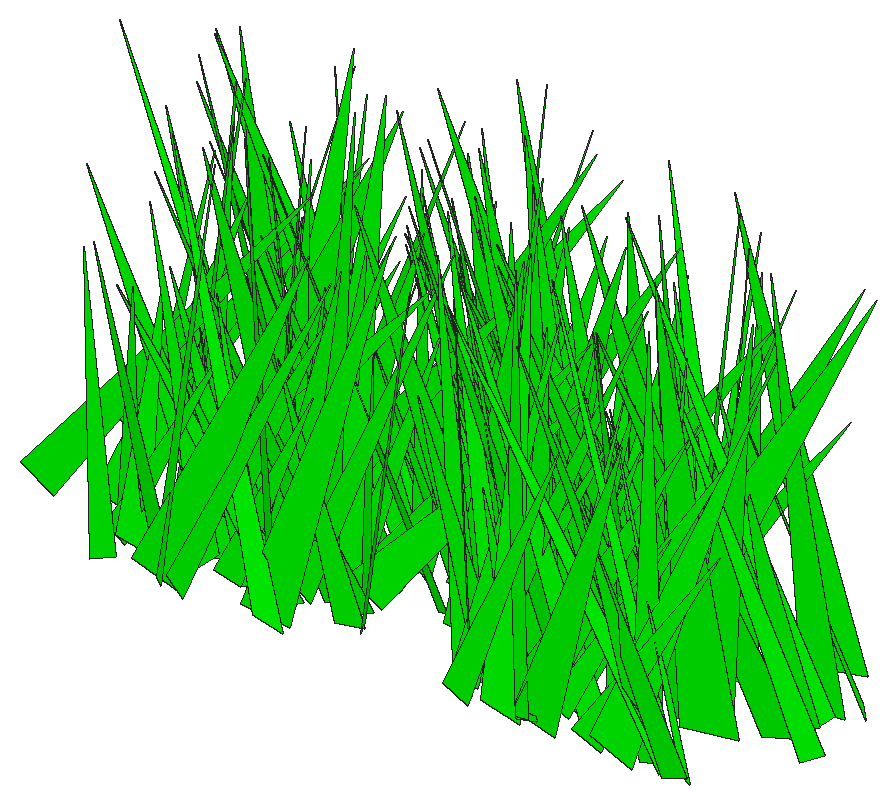
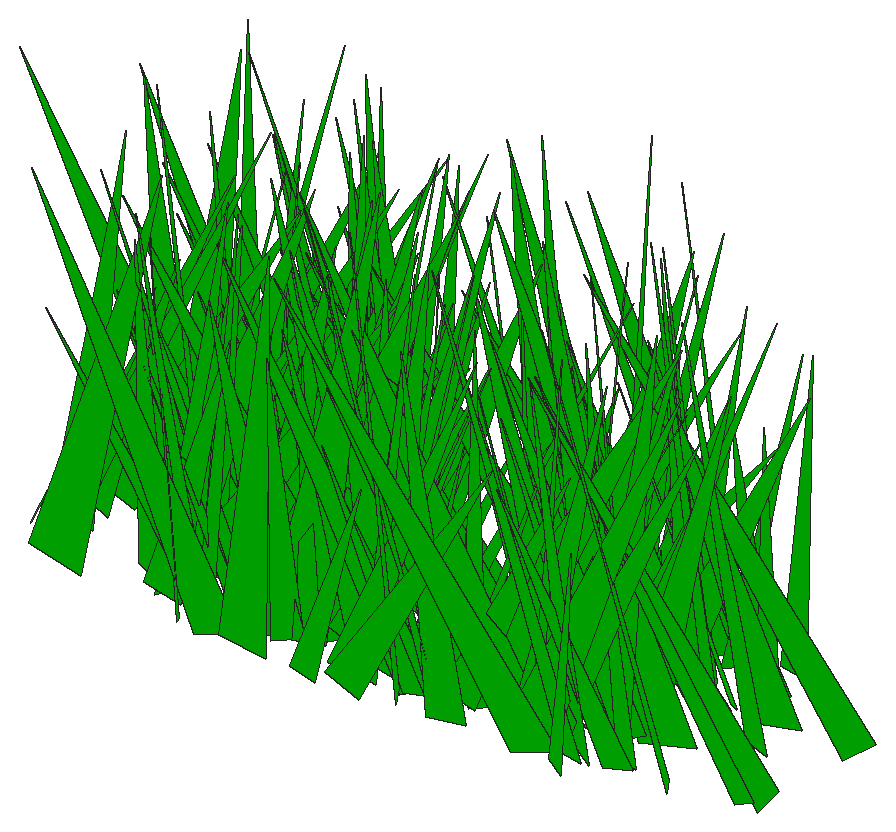
# SketchUp Ruby script. Lengths in inches.
U = 1.inch
M = Sketchup.active_model
def pt(a) = Geom::Point3d.new(a.map { |v| v * U })
def face(e, loops, mat)
  f = e.add_face(loops[0].map { |a| pt(a) })
  loops[1..].each { |l| e.add_face(l.map { |a| pt(a) }).erase! }
  f.material = f.back_material = mat if mat
  f
end
# faces: each face lists its corners as indices into pts; further lists are holes
def faces(e, pts, list, mat = nil) = list.each { |f| face(e, (f[0].is_a?(Array) ? f : [f]).map { |l| l.map { |i| pts[i] } }, mat) }
# xy, xz, yz: faces in a plane at the given z, y or x. An outline is a flat list of corners, or four numbers for a rectangle; further outlines are holes
def ring(l) = l.size == 4 ? [[l[0], l[1]], [l[2], l[1]], [l[2], l[3]], [l[0], l[3]]] : l.each_slice(2).to_a
def flat(e, list, mat, &to3) = list.each { |f| face(e, (f[0].is_a?(Array) ? f : [f]).map { |l| ring(l).map { |u, v| to3.(u, v) } }, mat) }
def xy(e, z, list, mat = nil) = flat(e, list, mat) { |x, y| [x, y, z] }
def xz(e, y, list, mat = nil) = flat(e, list, mat) { |x, z| [x, y, z] }
def yz(e, x, list, mat = nil) = flat(e, list, mat) { |y, z| [x, y, z] }
def lines(e, pts, list) = list.each { |a, b| e.add_line(pt(pts[a]), pt(pts[b])) }
# prism: a flat outline (further loops are holes) pulled along v
def prism(e, loops, v, mat = nil)
  f = face(e, loops, mat); d = Geom::Vector3d.new(v.map { |x| x * U })
  f.pushpull(f.normal.samedirection?(d) ? d.length : -d.length)
end
def box(e, o, s, mat = nil) = prism(e, [[o, [o[0] + s[0], o[1], o[2]], [o[0] + s[0], o[1] + s[1], o[2]], [o[0], o[1] + s[1], o[2]]]], [0, 0, s[2]], mat)
def at(x, y, z, deg = 0) = Geom::Transformation.translation(pt([x, y, z])) * Geom::Transformation.rotation(ORIGIN, Z_AXIS, deg.degrees)
def axes(o, x, y, z) = Geom::Transformation.new([*x, 0, *y, 0, *z, 0, *pt(o).to_a, 1])
def part(name) = M.definitions.add(name)
# library, detail: a bought-in or finely detailed component or shape, given as its bounding box
def library(name, o, s) = part(name).tap { |d| box(d.entities, o, s) }
def detail(e, o, s) = box(e.add_group.entities, o, s)
def put(e, d, t, mat = nil) = e.add_instance(d, t).tap { |i| i.material = mat if mat }
def group(e, t, mat = nil) = e.add_group.tap { |g| g.transformation = t; g.material = mat if mat }.entities
root = M.entities
M.materials.add("[0065_Lime]").color = [0, 255, 0]
c1 = part("fur_instance\#9")
p = [[0.8125,0,1.79],[0.67,-0.02,1.48],[0,-0.11,0],[0,0.11,0]]
faces(c1.entities,p,[[0,1,2,3]])
put(root,c1,axes([27.24,22.38,1.48],[7.31174,-0.39433,0.70196],[2.47884,1.00353,1.80658],[-1.57323,-0.25146,6.10893]),"[0065_Lime]")
put(root,c1,axes([31.46,23.04,1.48],[-8.52784,0.29529,1.08931],[-2.31792,-1.1863,-1.2302],[0.91482,-0.25308,7.03745]),"[0065_Lime]")
put(root,c1,axes([29,18.58,1.48],[4.59587,-0.53005,1.40933],[3.49281,0.69007,1.16069],[-2.24308,-0.01149,4.69495]),"[0065_Lime]")
put(root,c1,axes([30.38,23.19,1.48],[2.12919,0.84974,2.51321],[-6.24961,0.42319,-1.29142],[-2.65654,-0.31451,5.05242]),"[0065_Lime]")
put(root,c1,axes([28.63,20.14,1.48],[-3.00897,-0.60409,0.65925],[4.0362,-0.43666,-1.21885],[1.68757,-0.03275,4.09063]),"[0065_Lime]")
put(root,c1,axes([25.1875,24.44,1.48],[7.63571,-0.36238,0.53307],[2.54655,0.91406,-3.31261],[0.77165,0.56939,5.65715]),"[0065_Lime]")
put(root,c1,axes([31.65,20.61,1.48],[-3.71065,0.80647,0.71768],[-5.70109,-0.47805,-1.50216],[-1.10248,-0.2423,5.35235]),"[0065_Lime]")
put(root,c1,axes([25.62,24.91,1.48],[6.39063,0.54386,0.13874],[-3.71413,0.84691,1.9469],[1.10205,-0.29952,5.75696]),"[0065_Lime]")
put(root,c1,axes([32,25.42,1.48],[-3.76719,-0.84383,1.15865],[6.05294,-0.45934,1.81138],[-1.20548,0.33059,5.47439]),"[0065_Lime]")
put(root,c1,axes([29.14,19.64,1.48],[-2.3727,0.69246,0.37677],[-4.74423,-0.33875,1.09419],[1.41112,0.02545,4.31221]),"[0065_Lime]")
put(root,c1,axes([24.97,20.83,1.48],[7.30915,-0.65946,0.64194],[4.44222,0.87253,-3.43001],[1.70712,0.55304,6.17696]),"[0065_Lime]")
put(root,c1,axes([27.48,21.08,1.48],[0.90145,0.99524,0.70755],[-6.89263,0.08955,1.58951],[1.84718,-0.15155,5.58583]),"[0065_Lime]")
put(root,c1,axes([30.6,24.53,1.48],[3.62891,0.99697,2.27573],[-7.10396,0.60027,-1.31666],[-2.77481,-0.23294,6.34708]),"[0065_Lime]")
put(root,c1,axes([30.47,19.35,1.48],[-5.55156,-0.60914,0.08606],[4.02373,-0.73265,-2.03309],[1.61643,-0.2683,5.35647]),"[0065_Lime]")
put(root,c1,axes([32.46,25.47,1.48],[-4.3204,0.97206,0.76351],[-6.89822,-0.57061,-1.48346],[-1.07243,-0.24569,6.46621]),"[0065_Lime]")
put(root,c1,axes([27.8,25.44,1.48],[8.165,0.11966,1.13344],[-0.60132,1.14853,-1.19703],[-1.51831,0.18863,6.56937]),"[0065_Lime]")
put(root,c1,axes([28.43,22.59,1.48],[8.64399,-0.23036,1.70844],[1.147,1.22609,1.69991],[-2.40484,-0.24321,6.95164]),"[0065_Lime]")
put(root,c1,axes([29.45,25.125,1.48],[4.98083,-0.36586,0.65326],[2.32801,0.69361,1.27264],[-1.41576,-0.1466,4.39091]),"[0065_Lime]")
put(root,c1,axes([28.45,19.81,1.48],[3.81867,0.42883,0.98629],[-3.24796,0.45472,1.69548],[0.48393,-0.33195,3.59661]),"[0065_Lime]")
put(root,c1,axes([30.4,21.1,1.48],[6.9537,0.81374,1.27128],[-5.20212,0.98555,-2.31197],[-2.98602,0.17802,6.9883]),"[0065_Lime]")
put(root,c1,axes([31.3,20.12,1.48],[6.27949,-0.5717,1.66336],[2.93161,0.88212,2.83688],[-3.48431,-0.28814,5.38462]),"[0065_Lime]")
put(root,c1,axes([32.28,23.26,1.48],[-8.15919,-0.59671,0.88702],[3.90599,-1.13637,-1.84377],[1.99129,-0.21595,7.25112]),"[0065_Lime]")
put(root,c1,axes([30.79,26.47,1.48],[4.05133,-0.3067,0.66427],[1.45987,0.5134,2.05196],[-1.81647,-0.27143,3.13068]),"[0065_Lime]")
put(root,c1,axes([30.11,20.57,1.48],[7.8765,0.09932,2.19649],[-0.23858,1.15576,-1.18509],[-2.78109,0.18213,6.32248]),"[0065_Lime]")
put(root,c1,axes([32.36,22.14,1.48],[-3.61363,0.35537,0.74914],[-2.69143,-0.47598,-1.02391],[-0.01415,-0.21916,3.43849]),"[0065_Lime]")
put(root,c1,axes([29.12,20.96,1.48],[5.68958,-0.04407,0.13112],[0.27234,0.78178,0.98569],[-0.224,-0.16887,4.52898]),"[0065_Lime]")
put(root,c1,axes([31,25.3125,1.48],[6.60297,0.74035,0.46292],[-4.57086,0.8603,-2.9672],[-2.68159,0.35658,6.19756]),"[0065_Lime]")
put(root,c1,axes([29.42,25.52,1.48],[1.57397,0.67962,0.31538],[-4.63986,0.19407,1.3076],[1.41924,-0.11926,3.92512]),"[0065_Lime]")
put(root,c1,axes([32.07,20.42,1.48],[-4.06736,-0.10484,1.09489],[1.15393,-0.5614,1.03489],[1.01831,0.2174,3.20049]),"[0065_Lime]")
put(root,c1,axes([34.87,24.59,1.48],[-4.96476,0.99746,1.25521],[-7.07895,-0.60537,-2.40567],[-1.63042,-0.40895,6.62273]),"[0065_Lime]")
put(root,c1,axes([34.44,19.68,1.48],[-3.46979,0.62478,0.16593],[-4.0987,-0.43434,-1.9071],[-1.73542,-0.22337,4.17241]),"[0065_Lime]")
put(root,c1,axes([34.42,23.29,1.48],[-7.19379,-0.06708,0.09262],[0.49066,-0.97855,1.46741],[-0.00946,0.254,5.67783]),"[0065_Lime]")
put(root,c1,axes([32.67,25.28,1.48],[-5.43603,0.49974,2.45261],[-4.5128,-0.72754,-1.65049],[1.17224,-0.4834,5.01957]),"[0065_Lime]")
put(root,c1,axes([32.43,25.25,1.48],[7.00593,0.4856,2.47902],[-2.13062,1.03245,-2.79288],[-4.0855,0.29429,5.70761]),"[0065_Lime]")
put(root,c1,axes([33.26,19.85,1.48],[-2.34254,0.7207,0.59506],[-5.12688,-0.30624,-0.92509],[-0.74549,-0.15853,4.49218]),"[0065_Lime]")
put(root,c1,axes([32.74,21.97,1.48],[-4.70993,0.23093,0.59338],[-1.43956,-0.65652,1.0013],[1.07733,0.13233,3.93215]),"[0065_Lime]")
put(root,c1,axes([32.06,24.22,1.48],[-3.78011,-0.39336,0.58553],[2.51547,-0.52972,-1.18008],[1.42373,-0.10847,3.63959]),"[0065_Lime]")
put(root,c1,axes([30.74,18.69,1.48],[7.93736,0.22721,2.24613],[-2.16637,1.14531,1.18305],[-2.3551,-0.28777,6.48188]),"[0065_Lime]")
put(root,c1,axes([29.86,25.22,1.48],[4.81076,0.44759,1.44128],[-3.6437,0.57975,2.0139],[0.0954,-0.42761,4.23909]),"[0065_Lime]")
put(root,c1,axes([31.04,23.62,1.48],[-1.81036,1.27367,1.27731],[-9.01104,-0.29078,1.26561],[1.85082,-0.16986,7.41122]),"[0065_Lime]")
put(root,c1,axes([32,22.7,1.48],[4.61273,0.80516,0.81269],[-5.45717,0.66109,-1.45344],[-2.01241,0.05281,5.80419]),"[0065_Lime]")
put(root,c1,axes([33.73,20.03,1.48],[0.64125,-0.62776,0.59127],[4.02991,0.12615,1.59639],[-2.06071,0.05136,3.30588]),"[0065_Lime]")
put(root,c1,axes([29.18,23.7,1.48],[3.6009,-1.21002,0.8703],[8.47054,0.45484,-1.99834],[1.88317,0.26787,7.32444]),"[0065_Lime]")
put(root,c1,axes([35.4,20.51,1.48],[-6.07148,-0.63604,0.35972],[4.50379,-0.82645,1.32929],[-0.63224,0.22068,6.01489]),"[0065_Lime]")
put(root,c1,axes([32.1,21.78,1.48],[-7.56677,0.10738,3.03402],[0.73364,-1.1031,2.51875],[3.73611,0.43408,5.65023]),"[0065_Lime]")
put(root,c1,axes([32.76,20.24,1.48],[3.63636,-0.17101,1.37041],[0.25971,0.51074,1.67966],[-2.06204,-0.23724,2.62823]),"[0065_Lime]")
put(root,c1,axes([30.19,23.97,1.48],[6.06021,-0.46769,1.11053],[3.59327,0.80516,-1.61137],[-0.17445,0.33718,5.3882]),"[0065_Lime]")
put(root,c1,axes([34.64,18.52,1.48],[-8.09068,0.5651,0.45602],[-3.78052,-1.11245,1.81487],[1.4815,0.24731,7.12161]),"[0065_Lime]")
put(root,c1,axes([34.35,21.02,1.48],[0.77309,-1.23959,0.12733],[8.57589,0.11076,1.68193],[-2.07345,-0.00406,7.00399]),"[0065_Lime]")
put(root,c1,axes([33.44,19.65,1.48],[-4.9149,0.24413,1.83922],[-2.36952,-0.70189,-1.06758],[1.58637,-0.29202,4.10368]),"[0065_Lime]")
put(root,c1,axes([33.26,22.09,1.48],[-7.80588,-0.30689,2.05938],[1.01437,-1.07831,-2.84054],[3.18601,-0.40857,5.94996]),"[0065_Lime]")
put(root,c1,axes([35,23.05,1.48],[-3.42222,-0.65458,0.48968],[4.64295,-0.45558,1.0622],[-0.71087,0.17564,4.58019]),"[0065_Lime]")
put(root,c1,axes([30.7,20.7,1.48],[2.81269,-0.74102,0.40694],[5.14305,0.36296,-1.37274],[1.26841,0.17149,4.66368]),"[0065_Lime]")
put(root,c1,axes([35.09,25.21,1.48],[-1.79234,0.70766,0.99132],[-4.99689,-0.18813,-1.47738],[-1.37072,-0.23951,4.08947]),"[0065_Lime]")
put(root,c1,axes([30.75,25.83,1.48],[8.38971,-0.28534,0.46525],[1.90486,1.16624,1.24072],[-0.90679,-0.19017,6.91086]),"[0065_Lime]")
put(root,c1,axes([32.0625,21.48,1.48],[-3.36593,0.64664,1.28953],[-3.78762,-0.51809,2.16426],[3.05679,0.07008,4.10164]),"[0065_Lime]")
put(root,c1,axes([32.76,21.9375,1.48],[-3.55119,-0.59167,1.40943],[3.85319,-0.55502,-1.38384],[2.42582,0.01545,4.26138]),"[0065_Lime]")
put(root,c1,axes([30.73,18.72,1.48],[0.6966,-1.13401,1.07496],[7.68457,0.02703,-2.33927],[2.79686,0.20817,6.15959]),"[0065_Lime]")
put(root,c1,axes([29.28,21.65,1.48],[4.05134,0.88781,0.72507],[-5.68072,0.4343,3.18205],[2.90562,-0.38879,5.21019]),"[0065_Lime]")
put(root,c1,axes([32.26,19.78,1.48],[1.63236,-0.57647,0.58851],[4.05108,0.19422,-1.05954],[0.97086,0.15883,3.43162]),"[0065_Lime]")
put(root,c1,axes([32.22,24.37,1.48],[5.73566,-0.1439,0.41558],[0.83523,0.77716,1.39029],[-0.7824,-0.22528,4.53073]),"[0065_Lime]")
put(root,c1,axes([34.33,19.15,1.48],[8.27058,0.12873,3.67062],[-2.34781,1.23927,2.04372],[-3.96117,-0.46574,6.45263]),"[0065_Lime]")
put(root,c1,axes([31.28,18.66,1.48],[6.64813,0.53494,1.43953],[-4.19276,0.82237,2.57124],[0.21324,-0.50818,5.67632]),"[0065_Lime]")
put(root,c1,axes([36.32,20.58,1.48],[-3.00258,-0.41802,0.26218],[2.83445,-0.37677,1.34786],[-0.95901,0.19521,3.16287]),"[0065_Lime]")
put(root,c1,axes([33.28,20.65,1.48],[-0.06196,-0.90183,1.36953],[6.49252,-0.05703,-1.06399],[1.36816,0.22978,5.1111]),"[0065_Lime]")
put(root,c1,axes([35.7,24.1,1.48],[-4.70782,0.03814,0.87173],[-0.6939,-0.61476,-1.57809],[0.86065,-0.287,3.4961]),"[0065_Lime]")
put(root,c1,axes([33.7,22.19,1.48],[-1.936,-0.90176,1.04675],[6.26825,-0.30972,-1.27006],[1.88361,0.10383,5.30237]),"[0065_Lime]")
put(root,c1,axes([37.9,21.88,1.48],[-7.69705,-0.29198,0.29811],[2.10916,-1.07001,0.914],[0.05713,0.16589,6.42027]),"[0065_Lime]")
put(root,c1,axes([33.02,19.88,1.48],[6.88446,0.19712,0.505],[-1.12008,0.91997,-1.93019],[-1.04823,0.3116,5.37917]),"[0065_Lime]")
put(root,c1,axes([34.2,21.69,1.48],[-2.10637,1.236,2.23685],[-9.03041,-0.35594,0.96409],[1.83965,-0.33201,7.29366]),"[0065_Lime]")
put(root,c1,axes([33.24,22.75,1.48],[3.38714,-0.85288,1.06915],[6.19585,0.44979,-0.96411],[0.42222,0.24152,5.57096]),"[0065_Lime]")
put(root,c1,axes([34.39,21.06,1.48],[6.86662,0.71639,3.21811],[-6.01518,1.00453,0.99876],[-2.33711,-0.4806,6.88451]),"[0065_Lime]")
put(root,c1,axes([36.41,19.81,1.48],[-0.62911,-0.63991,1.08982],[4.63821,-0.04245,0.93635],[-1.01024,0.20361,3.6203]),"[0065_Lime]")
put(root,c1,axes([35.74,21.29,1.48],[7.47327,0.53315,1.76455],[-2.21384,0.9824,-3.74273],[-3.76836,0.48017,5.69818]),"[0065_Lime]")
put(root,c1,axes([36.03,23.34,1.48],[6.73913,0.79277,0.67794],[-4.31233,0.827,-4.04313],[-3.73207,0.47596,5.89594]),"[0065_Lime]")
put(root,c1,axes([37.95,26.56,1.48],[-0.57662,-0.79796,0.598],[5.19884,-0.02944,2.00061],[-2.40013,0.12795,4.18977]),"[0065_Lime]")
put(root,c1,axes([34.6,26.34,1.48],[-1.28453,-0.92384,0.95227],[6.46428,-0.21406,-1.18929],[1.67579,0.11757,5.31756]),"[0065_Lime]")
put(root,c1,axes([31.73,26.18,1.48],[3.05563,1.15514,0.0185],[-7.54446,0.3927,2.83958],[3.26495,-0.17366,6.54423]),"[0065_Lime]")
put(root,c1,axes([31.77,22.54,1.48],[3.23221,-0.94446,1.44478],[6.17309,0.26332,-3.36941],[3.19737,0.44636,5.04472]),"[0065_Lime]")
put(root,c1,axes([38.33,26.04,1.48],[-5.02287,-0.71257,0.95099],[5.20003,-0.67822,1.14335],[-0.20533,0.25528,5.69209]),"[0065_Lime]")
put(root,c1,axes([34.8,21.95,1.48],[4.35896,-0.42854,1.1615],[3.3495,0.58562,-1.07677],[-0.34747,0.26922,4.19117]),"[0065_Lime]")
put(root,c1,axes([36.93,24.91,1.48],[-4.01383,-0.40934,0.21134],[2.71355,-0.54436,-1.23184],[1.09097,-0.15204,3.84147]),"[0065_Lime]")
put(root,c1,axes([34.32,18.83,1.48],[4.55432,-0.95925,1.35246],[7.01581,0.6058,-1.23355],[0.38029,0.31167,6.56015]),"[0065_Lime]")
put(root,c1,axes([32.66,25.37,1.48],[6.84505,-0.88791,0.30615],[6.19986,0.92468,-1.85185],[1.27735,0.27004,7.34777]),"[0065_Lime]")
put(root,c1,axes([38.4375,22.28,1.48],[-3.7554,-0.36263,0.77595],[2.74661,-0.48085,1.2651],[-0.16095,0.25538,3.48382]),"[0065_Lime]")
put(root,c1,axes([34.23,20.41,1.48],[6.90659,0.55604,1.07512],[-4.16845,0.93448,1.52274],[-0.1713,-0.32111,6.29304]),"[0065_Lime]")
put(root,c1,axes([34.28,25.18,1.48],[2.8761,0.66224,0.83559],[-4.53985,0.31487,1.97694],[1.62973,-0.29159,4.03242]),"[0065_Lime]")
put(root,c1,axes([37.59,25.9,1.48],[-7.39528,0.13923,2.40911],[-1.65613,-1.08179,-1.26864],[2.64781,-0.28775,5.9351]),"[0065_Lime]")
put(root,c1,axes([36.42,26.12,1.48],[8.31067,0.16513,2.38382],[-0.60758,1.22146,-1.43371],[-3.09846,0.20338,6.67502]),"[0065_Lime]")
put(root,c1,axes([37.85,25.12,1.48],[-6.1838,-0.66036,0.47822],[4.29819,-0.83955,-2.07369],[1.98911,-0.23881,5.96767]),"[0065_Lime]")
put(root,c1,axes([37.63,25.28,1.48],[4.07699,-0.9895,1.08281],[6.75053,0.6025,1.63239],[-2.40623,0.01371,6.41422]),"[0065_Lime]")
put(root,c1,axes([39.42,22.9,1.48],[-6.94626,-0.01756,0.77063],[0.58219,-0.85237,2.8212],[0.75779,0.49387,4.8965]),"[0065_Lime]")
put(root,c1,axes([39.49,24.54,1.48],[-3.32818,-0.70735,0.54631],[4.9953,-0.43563,1.23452],[-0.91533,0.19454,4.75086]),"[0065_Lime]")
put(root,c1,axes([39.5,22.09,1.48],[-0.92688,-1.08023,0.89166],[7.50309,-0.08462,1.72531],[-2.00062,0.18311,6.05746]),"[0065_Lime]")
put(root,c1,axes([35.125,26.12,1.48],[8.46546,0.27052,1.33272],[-2.19824,1.18506,1.17822],[-1.24837,-0.25231,6.96274]),"[0065_Lime]")
put(root,c1,axes([38.71,23.54,1.48],[-7.23871,-0.05482,1.49299],[0.04202,-1.0323,-1.13529],[1.87599,-0.1884,5.78628]),"[0065_Lime]")
put(root,c1,axes([36.28,23.09,1.48],[5.68248,-0.03481,1.22168],[0.85153,0.74876,-1.90566],[-1.26176,0.34854,4.21591]),"[0065_Lime]")
put(root,c1,axes([39.49,22.79,1.48],[-6.30534,-0.84975,1.88278],[6.43525,-0.87268,1.06135],[0.71748,0.3595,7.0267]),"[0065_Lime]")
put(root,c1,axes([38.09,23.95,1.48],[-4.2405,-0.1173,0.95165],[0.31347,-0.57531,-1.4521],[1.40265,-0.22607,3.20157]),"[0065_Lime]")
put(root,c1,axes([36.76,19.91,1.48],[6.71529,-0.01641,1.65695],[-0.24113,0.97131,0.96898],[-2.02609,-0.17,5.37652]),"[0065_Lime]")
put(root,c1,axes([36.18,25.74,1.48],[2.37602,0.50035,0.64965],[-3.59631,0.29832,1.00342],[0.61933,-0.18727,3.33428]),"[0065_Lime]")
put(root,c1,axes([39.62,22.52,1.48],[-5.90576,0.48933,1.51849],[-3.86602,-0.81303,-1.16919],[0.81567,-0.3106,5.4528]),"[0065_Lime]")
put(root,c1,axes([39.56,22.38,1.48],[2.0045,-0.56026,0.62481],[3.31699,0.29537,1.83414],[-2.34197,-0.06119,3.13251]),"[0065_Lime]")
put(root,c1,axes([37.45,23.15,1.48],[-0.8931,0.54885,0.82144],[-3.77686,-0.16484,0.97362],[1.41815,-0.09335,3.11028]),"[0065_Lime]")
put(root,c1,axes([39.15,26.73,1.48],[1.1823,-0.57354,0.11381],[3.83406,0.16292,1.15979],[-1.40695,-0.03798,3.25617]),"[0065_Lime]")
put(root,c1,axes([39.89,24.35,1.48],[1.59828,-1.04983,2.44419],[7.7575,0.31622,1.19505],[-2.16065,0.35878,6.09865]),"[0065_Lime]")
put(root,c1,axes([41.98,24.05,1.48],[-2.90564,1.22535,1.69969],[-8.7058,-0.31152,-2.32157],[-2.14894,-0.39481,7.10699]),"[0065_Lime]")
put(root,c1,axes([39.33,23.19,1.48],[2.44554,1.01832,0.22681],[-7.07337,0.34404,-1.29873],[-1.60102,0.03548,6.08428]),"[0065_Lime]")
put(root,c1,axes([38.125,24.25,1.48],[-1.48251,0.98538,1.0164],[-6.93887,-0.2403,1.10987],[1.60883,-0.12839,5.7235]),"[0065_Lime]")
put(root,c1,axes([35.375,22.39,1.48],[3.64267,-0.84643,0.59277],[5.57952,0.42035,-2.57281],[2.38415,0.3095,5.11537]),"[0065_Lime]")
put(root,c1,axes([35.59,21.46,1.48],[1.60231,0.88211,0.31295],[-5.36175,0.16242,2.82227],[3.28745,-0.16503,4.45053]),"[0065_Lime]")
put(root,c1,axes([40.79,24.92,1.48],[0.23717,1.27318,2.00415],[-9.19822,0.10108,-1.43158],[-1.88646,-0.33281,7.23225]),"[0065_Lime]")
put(root,c1,axes([41.71,23.41,1.48],[-8.65989,-0.49796,0.41819],[3.3773,-1.19864,-1.55316],[1.19006,-0.22191,7.45087]),"[0065_Lime]")
put(root,c1,axes([36.14,25.54,1.48],[5.628,-0.75243,0.83215],[5.30431,0.70811,-2.28092],[1.25837,0.38034,5.89283]),"[0065_Lime]")
put(root,c1,axes([38.11,23.99,1.48],[-0.34736,1.08524,0.44784],[-7.51623,-0.06586,1.49044],[1.85914,-0.06349,6.10928]),"[0065_Lime]")
put(root,c1,axes([42.5625,22.58,1.48],[-4.37768,-0.56495,0.31656],[3.84625,-0.55839,1.79974],[-1.23381,0.26381,4.48729]),"[0065_Lime]")
put(root,c1,axes([38.22,25.04,1.48],[-1.29081,0.71333,2.13496],[-5.26444,-0.29555,1.203],[2.22372,-0.28561,4.08727]),"[0065_Lime]")
put(root,c1,axes([39.98,20.34,1.48],[6.17672,-0.61391,2.02845],[3.94612,0.93545,1.53656],[-3.12003,-0.03223,5.95911]),"[0065_Lime]")
put(root,c1,axes([40.9,23.77,1.48],[1.04183,1.237,1.112],[-8.73088,0.18022,-1.30573],[-1.77098,-0.16079,7.09137]),"[0065_Lime]")
put(root,c1,axes([43.3,24.21,1.48],[-3.40117,-0.7899,0.34607],[5.18596,-0.41102,2.28601],[-2.21049,0.25109,4.83068]),"[0065_Lime]")
put(root,c1,axes([41.35,19.76,1.48],[1.1734,-0.71894,0.98522],[4.93579,0.21071,1.26291],[-1.81172,0.10842,4.07873]),"[0065_Lime]")
put(root,c1,axes([41.375,20.1,1.48],[6.27044,-0.36018,4.20306],[4.00823,1.04332,-0.96053],[-4.14779,0.46371,5.42579]),"[0065_Lime]")
put(root,c1,axes([39.0625,21.95,1.48],[7.3953,0.60919,2.62837],[-4.99877,1.06355,1.04569],[-2.06127,-0.39358,6.89403]),"[0065_Lime]")
put(root,c1,axes([41.92,22.54,1.48],[2.46873,-1.04619,2.21521],[7.3838,0.44934,1.66642],[-2.88581,0.25471,6.15885]),"[0065_Lime]")
put(root,c1,axes([42.35,23.43,1.48],[0.09975,-1.06518,0.98539],[7.32773,0.06395,1.82566],[-2.28795,0.15838,5.8901]),"[0065_Lime]")
put(root,c1,axes([42.18,24.79,1.48],[0.35253,-0.69612,1.99345],[5.09291,0.17497,1.45145],[-2.14713,0.30072,3.77007]),"[0065_Lime]")
put(root,c1,axes([40.14,25.23,1.48],[-3.27967,-0.60621,0.76806],[4.00412,-0.4779,-1.32668],[1.86292,-0.04006,4.20369]),"[0065_Lime]")
put(root,c1,axes([39.28,21.36,1.48],[0.34822,-1.19056,0.47024],[8.40699,0.03683,-0.99473],[1.20123,0.08739,6.8255]),"[0065_Lime]")
put(root,c1,axes([41.64,23.65,1.48],[-5.23945,-0.04602,0.85845],[-0.08708,-0.6992,-1.6076],[1.10158,-0.27415,3.95599]),"[0065_Lime]")
put(root,c1,axes([41.12,19.07,1.48],[-7.04194,0.05973,2.07122],[0.58299,-0.97588,2.2545],[2.51489,0.39348,5.27702]),"[0065_Lime]")
put(root,c1,axes([42.03,20.61,1.48],[-5.13777,0.25233,0.9931],[-2.05889,-0.70611,-1.03569],[0.69002,-0.22813,4.30418]),"[0065_Lime]")
put(root,c1,axes([40.6,25.54,1.48],[-3.91595,0.70211,0.21082],[-4.6708,-0.52958,1.69601],[1.79347,0.15381,4.87729]),"[0065_Lime]")
put(root,c1,axes([40.53,23.82,1.48],[-3.49945,-0.46349,0.24548],[2.80968,-0.44806,-1.84686],[1.75399,-0.20699,3.44821]),"[0065_Lime]")
put(root,c1,axes([38.93,24.15,1.48],[-0.09459,-1.18256,0.52723],[8.12885,-0.03729,-1.83791],[2.27307,0.08415,6.59459]),"[0065_Lime]")
put(root,c1,axes([41.89,20.53,1.48],[-7.68244,-0.11726,1.84664],[0.24863,-1.09493,-1.6453],[2.40593,-0.26126,6.0666]),"[0065_Lime]")
put(root,c1,axes([43.7,20.23,1.48],[-7.4598,-0.62589,0.84933],[4.56559,-1.03643,0.93878],[0.29263,0.2148,7.00465]),"[0065_Lime]")
put(root,c1,axes([40.24,23.02,1.48],[5.9463,0.5313,0.76187],[-3.51549,0.83541,-1.36765],[-1.67766,0.13254,5.56623]),"[0065_Lime]")
put(root,c1,axes([41.31,26.57,1.48],[3.33168,-0.98631,0.57311],[6.8598,0.47851,1.20967],[-1.64555,-0.00219,6.20313]),"[0065_Lime]")
put(root,c1,axes([41.92,21.18,1.48],[5.99274,1.00348,1.30366],[-6.47347,0.86254,-2.55883],[-3.41492,0.12592,7.1384]),"[0065_Lime]")
put(root,c1,axes([43,23.49,1.48],[1.85346,1.10334,0.60422],[-7.4571,0.28007,-2.00234],[-2.56846,-0.01694,6.24949]),"[0065_Lime]")
put(root,c1,axes([44.78,23.83,1.48],[-4.41568,0.81024,0.77949],[-5.59054,-0.53614,-2.27941],[-1.70661,-0.34012,5.45009]),"[0065_Lime]")
put(root,c1,axes([40.73,25.53,1.48],[-0.49479,0.97285,0.01368],[-6.80291,-0.06876,1.04766],[1.28588,0.01059,5.54786]),"[0065_Lime]")
put(root,c1,axes([41.04,23.42,1.48],[-0.66567,-0.68804,1.00397],[4.77491,-0.14268,-1.1818],[1.6428,0.13591,3.8418]),"[0065_Lime]")
put(root,c1,axes([40.66,19.3125,1.48],[6.74947,-0.44564,1.67777],[3.55495,0.94987,-1.00783],[-1.29416,0.28504,5.98167]),"[0065_Lime]")
put(root,c1,axes([43.16,18.71,1.48],[0.46587,0.59659,0.31652],[-4.10268,0.07769,-0.91165],[-1.15966,-0.0352,3.35243]),"[0065_Lime]")
put(root,c1,axes([44.55,19.93,1.48],[-7.23129,0.40844,1.46637],[-3.31112,-0.98447,-1.61514],[0.85737,-0.35708,6.13022]),"[0065_Lime]")
put(root,c1,axes([40.12,20.84,1.48],[4.54962,0.49898,0.61024],[-3.59218,0.59493,1.41871],[0.51842,-0.25666,4.475]),"[0065_Lime]")
put(root,c1,axes([41.87,20.66,1.48],[5.03008,-0.84405,0.35016],[5.80594,0.70063,1.40855],[-1.59919,-0.11123,6.21525]),"[0065_Lime]")
put(root,c1,axes([42.45,18.63,1.48],[-6.70509,0.80281,1.75154],[-5.16554,-0.98549,2.05245],[3.25502,0.0898,6.86516]),"[0065_Lime]")
put(root,c1,axes([42.84,18.72,1.48],[6.07755,0.72788,2.19712],[-5.06892,0.92931,-1.03935],[-2.90422,-0.09878,6.41186]),"[0065_Lime]")
put(root,c1,axes([40.89,18.66,1.48],[3.81698,0.55833,1.39415],[-4.31601,0.46802,1.53767],[0.31241,-0.35586,4.20965]),"[0065_Lime]")
put(root,c1,axes([43.4,23.28,1.48],[1.69351,-0.74762,0.05284],[5.1107,0.23122,1.24758],[-1.48055,-0.05701,4.36695]),"[0065_Lime]")
put(root,c1,axes([43.1,25.95,1.48],[-6.64899,-0.55008,1.59954],[3.47438,-0.96805,-1.59981],[2.66834,-0.11021,6.06881]),"[0065_Lime]")
put(root,c1,axes([41.52,22.1875,1.48],[-0.80101,0.5488,1.95754],[-4.14515,-0.23365,1.07273],[1.96533,-0.26913,3.06037]),"[0065_Lime]")
put(root,c1,axes([43.12,21.17,1.48],[3.87734,0.23731,0.9624],[-1.10861,0.53845,-1.49387],[-1.73865,0.18588,3.09876]),"[0065_Lime]")
put(root,c1,axes([39.38,24.42,1.48],[2.96488,-0.96768,1.65332],[6.54156,0.23663,-3.12063],[2.96038,0.44626,5.23983]),"[0065_Lime]")
put(root,c1,axes([44.68,25.35,1.48],[-7.80135,0.66883,0.58656],[-4.37324,-1.06527,2.21862],[2.01254,0.27783,7.09477]),"[0065_Lime]")
put(root,c1,axes([44.4,25.22,1.48],[-5.33301,0.62495,0.06259],[-4.25875,-0.72223,1.55885],[1.28429,0.20017,5.42911]),"[0065_Lime]")
put(root,c1,axes([44.78,25.63,1.48],[-0.1747,0.79574,0.91428],[-5.60863,0.01409,-1.11988],[-1.36932,-0.15922,4.47032]),"[0065_Lime]")
put(root,c1,axes([41.47,22.96,1.48],[2.02399,0.68555,0.67473],[-4.76046,0.23531,1.43686],[1.35206,-0.19775,4.04898]),"[0065_Lime]")
put(root,c1,axes([45.95,23.73,1.48],[-2.28774,-1.04874,2.32568],[7.82052,-0.20756,1.95365],[-1.64823,0.47082,6.04161]),"[0065_Lime]")
put(root,c1,axes([46.76,21.49,1.48],[-4.73326,-0.9415,0.19771],[6.5581,-0.64145,1.52362],[-1.39401,0.17909,6.49652]),"[0065_Lime]")
put(root,c1,axes([40.58,19.97,1.48],[7.97102,0.50073,1.14362],[-3.82192,1.0705,1.91917],[-0.26044,-0.3842,6.83793]),"[0065_Lime]")
put(root,c1,axes([45.65,22.87,1.48],[0.28212,0.6837,0.67029],[-4.51218,0.0827,-1.57021],[-1.99831,-0.09022,3.64016]),"[0065_Lime]")
put(root,c1,axes([42,25.68,1.48],[5.92885,-0.12351,0.51986],[1.00601,0.81215,-1.12572],[-0.41102,0.20627,4.74357]),"[0065_Lime]")
put(root,c1,axes([43.47,25.68,1.48],[-7.09703,0.3738,2.61825],[-1.1712,-1.03429,2.84757],[4.00822,0.35964,5.46799]),"[0065_Lime]")
put(root,c1,axes([43.56,26.51,1.48],[-6.42147,-0.24756,2.76647],[1.15215,-1.01456,-1.27273],[3.65288,-0.11518,5.26466]),"[0065_Lime]")
put(root,c1,axes([47.84,19.02,1.48],[-7.92345,0.31681,0.18024],[-2.22352,-1.06582,-1.89679],[-0.43402,-0.32345,6.42682]),"[0065_Lime]")
put(root,c1,axes([45.21,23.43,1.48],[0.25728,1.01962,0.67546],[-7.21013,0.05407,-0.91812],[-1.16444,-0.10954,5.83419]),"[0065_Lime]")
put(root,c1,axes([44.79,21.15,1.48],[-6.70901,-0.10623,2.08988],[0.0395,-0.97761,-1.58123],[2.6779,-0.25172,5.25916]),"[0065_Lime]")
put(root,c1,axes([44.94,20.53,1.48],[1.79123,0.6215,0.2735],[-4.26641,0.25534,-0.95537],[-1.21366,0.01966,3.76209]),"[0065_Lime]")
put(root,c1,axes([43.06,24.57,1.48],[3.37749,0.47293,1.30684],[-3.72232,0.40867,1.40934],[0.23031,-0.33045,3.61333]),"[0065_Lime]")
put(root,c1,axes([43.73,18.85,1.48],[6.48126,-0.15251,1.51234],[1.4939,0.91537,-1.14286],[-1.55016,0.24451,5.22175]),"[0065_Lime]")
put(root,c1,axes([42.86,26.08,1.48],[4.60572,0.34229,0.59546],[-2.52618,0.59074,1.54902],[0.29673,-0.28364,3.94483]),"[0065_Lime]")
put(root,c1,axes([42.78,24.55,1.48],[7.81116,-0.05176,0.93339],[0.67021,1.06542,-1.73098],[-1.00164,0.3092,6.1207]),"[0065_Lime]")
put(root,c1,axes([45.39,20.8,1.48],[-7.6236,-0.74229,0.633],[4.23376,-0.95648,-3.84744],[3.25366,-0.49466,6.48958]),"[0065_Lime]")
put(root,c1,axes([43.5,18.73,1.48],[-0.41477,-0.94786,0.6129],[6.44606,-0.08823,-1.68582],[2.12545,0.0826,5.23235]),"[0065_Lime]")
put(root,c1,axes([45.36,25.19,1.48],[5.05697,0.86997,0.15868],[-5.70155,0.66758,-2.4216],[-2.4209,0.24501,6.03465]),"[0065_Lime]")
put(root,c1,axes([42.58,19.58,1.48],[1.77765,0.86348,1.7818],[-6.12094,0.11039,2.24783],[2.25694,-0.38073,4.69281]),"[0065_Lime]")
put(root,c1,axes([43.57,19.68,1.48],[2.42543,0.527,0.1665],[-3.63803,0.3211,1.00722],[0.93407,-0.11779,3.4906]),"[0065_Lime]")
put(root,c1,axes([42.26,26.47,1.48],[4.56461,-0.9428,0.53809],[6.55762,0.59479,-1.88511],[1.56589,0.25744,6.3259]),"[0065_Lime]")
put(root,c1,axes([48.26,18.74,1.48],[-5.93578,-0.62295,1.04627],[4.6031,-0.77673,1.78174],[-0.34587,0.35362,5.75682]),"[0065_Lime]")
put(root,c1,axes([42.82,26.01,1.48],[3.28785,0.62294,0.38611],[-4.16154,0.39903,1.87368],[1.60005,-0.24221,4.07983]),"[0065_Lime]")
put(root,c1,axes([45.12,23.21,1.48],[8.67676,0.14781,2.52367],[-0.11511,1.24724,-2.18589],[-3.27401,0.34786,6.76508]),"[0065_Lime]")
put(root,c1,axes([47.63,19.26,1.48],[-8.79445,0.02744,1.79472],[-0.80241,-1.22265,-1.97518],[2.06458,-0.35831,6.87726]),"[0065_Lime]")
put(root,c1,axes([43.27,20.2,1.48],[3.91675,0.7321,0.3809],[-5.03851,0.50589,1.69783],[1.40614,-0.22653,5.0227]),"[0065_Lime]")
put(root,c1,axes([49.15,22.22,1.48],[-2.41465,-0.98223,0.38122],[6.64359,-0.29893,2.03322],[-2.22335,0.1735,5.66145]),"[0065_Lime]")
put(root,c1,axes([48.15,25.98,1.48],[0.01387,1.1301,2.19857],[-8.20686,0.09814,-1.65621],[-2.15254,-0.36691,6.32869]),"[0065_Lime]")
put(root,c1,axes([47.38,19.04,1.48],[0.40064,-0.68805,0.40279],[4.72335,0.07337,1.09096],[-1.38237,0.05127,3.84439]),"[0065_Lime]")
put(root,c1,axes([49.49,23.52,1.48],[-8.80058,0.30758,1.01795],[-2.47694,-1.17398,-2.28221],[0.47125,-0.42658,7.01469]),"[0065_Lime]")
put(root,c1,axes([45.62,21.14,1.48],[6.98273,-0.29718,1.54035],[1.677,1.00191,1.44729],[-2.29051,-0.17241,5.75546]),"[0065_Lime]")
put(root,c1,axes([47.46,21.21,1.48],[1.79657,-1.2621,0.46232],[8.8892,0.26158,1.07314],[-1.40648,0.04107,7.37296]),"[0065_Lime]")
put(root,c1,axes([48.53,18.86,1.48],[-6.54796,0.13187,0.88281],[-0.6092,-0.90062,1.51835],[1.29904,0.24236,5.16194]),"[0065_Lime]")
put(root,c1,axes([46.86,19.32,1.48],[6.96921,-0.69321,1.60743],[4.52089,1.01407,1.68536],[-2.79348,-0.08828,6.73778]),"[0065_Lime]")
put(root,c1,axes([45.17,18.87,1.48],[0.62911,0.66887,0.97185],[-4.41438,0.00316,1.81779],[2.1445,-0.18971,3.45674]),"[0065_Lime]")
put(root,c1,axes([43.79,23.23,1.48],[-0.55447,1.22452,2.5984],[-8.16564,-0.27812,3.23909],[4.41217,-0.36084,6.32116]),"[0065_Lime]")
put(root,c1,axes([49.26,23,1.48],[2.06413,0.79676,1.10775],[-5.08158,0.34534,-2.05839],[-2.86062,-0.03855,4.45583]),"[0065_Lime]")
put(root,c1,axes([46.76,22.03,1.48],[-1.15812,-1.09469,1.64101],[7.89057,-0.21074,-1.02627],[1.58108,0.24987,6.32375]),"[0065_Lime]")
put(root,c1,axes([50.47,21.83,1.48],[-6.47511,0.39801,0.92861],[-3.04779,-0.86588,-1.62535],[0.19207,-0.32225,5.51425]),"[0065_Lime]")
put(root,c1,axes([49.96,24.67,1.48],[-5.71504,-0.16688,0.10052],[1.07153,-0.75429,-1.65199],[0.52673,-0.27616,4.45133]),"[0065_Lime]")
put(root,c1,axes([46.06,18.79,1.48],[-3.8545,0.99401,1.42834],[-6.0276,-0.59165,3.03486],[4.09779,0.06471,5.80763]),"[0065_Lime]")
put(root,c1,axes([49.21,23.91,1.48],[3.4424,0.91835,2.47056],[-6.68188,0.58391,-1.11301],[-2.69996,-0.27419,5.9044]),"[0065_Lime]")
